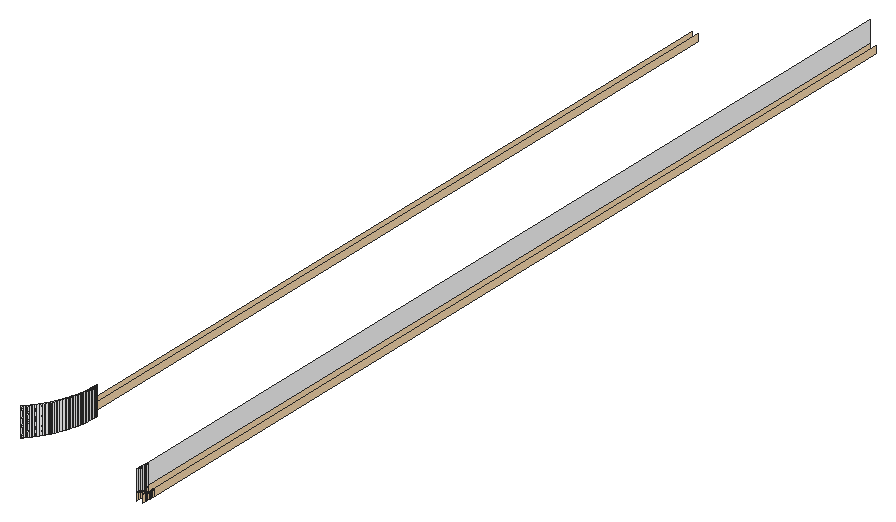
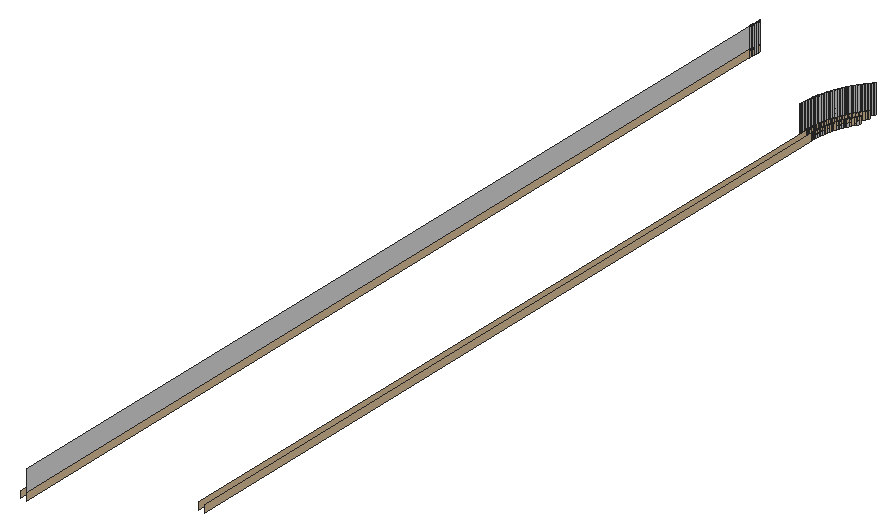
# SketchUp Ruby script. Lengths in inches.
U = 1.inch
M = Sketchup.active_model
def pt(a) = Geom::Point3d.new(a.map { |v| v * U })
def face(e, loops, mat)
  f = e.add_face(loops[0].map { |a| pt(a) })
  loops[1..].each { |l| e.add_face(l.map { |a| pt(a) }).erase! }
  f.material = f.back_material = mat if mat
  f
end
# faces: each face lists its corners as indices into pts; further lists are holes
def faces(e, pts, list, mat = nil) = list.each { |f| face(e, (f[0].is_a?(Array) ? f : [f]).map { |l| l.map { |i| pts[i] } }, mat) }
# xy, xz, yz: faces in a plane at the given z, y or x. An outline is a flat list of corners, or four numbers for a rectangle; further outlines are holes
def ring(l) = l.size == 4 ? [[l[0], l[1]], [l[2], l[1]], [l[2], l[3]], [l[0], l[3]]] : l.each_slice(2).to_a
def flat(e, list, mat, &to3) = list.each { |f| face(e, (f[0].is_a?(Array) ? f : [f]).map { |l| ring(l).map { |u, v| to3.(u, v) } }, mat) }
def xy(e, z, list, mat = nil) = flat(e, list, mat) { |x, y| [x, y, z] }
def xz(e, y, list, mat = nil) = flat(e, list, mat) { |x, z| [x, y, z] }
def yz(e, x, list, mat = nil) = flat(e, list, mat) { |y, z| [x, y, z] }
def lines(e, pts, list) = list.each { |a, b| e.add_line(pt(pts[a]), pt(pts[b])) }
# prism: a flat outline (further loops are holes) pulled along v
def prism(e, loops, v, mat = nil)
  f = face(e, loops, mat); d = Geom::Vector3d.new(v.map { |x| x * U })
  f.pushpull(f.normal.samedirection?(d) ? d.length : -d.length)
end
def box(e, o, s, mat = nil) = prism(e, [[o, [o[0] + s[0], o[1], o[2]], [o[0] + s[0], o[1] + s[1], o[2]], [o[0], o[1] + s[1], o[2]]]], [0, 0, s[2]], mat)
def at(x, y, z, deg = 0) = Geom::Transformation.translation(pt([x, y, z])) * Geom::Transformation.rotation(ORIGIN, Z_AXIS, deg.degrees)
def axes(o, x, y, z) = Geom::Transformation.new([*x, 0, *y, 0, *z, 0, *pt(o).to_a, 1])
def part(name) = M.definitions.add(name)
# library, detail: a bought-in or finely detailed component or shape, given as its bounding box
def library(name, o, s) = part(name).tap { |d| box(d.entities, o, s) }
def detail(e, o, s) = box(e.add_group.entities, o, s)
def put(e, d, t, mat = nil) = e.add_instance(d, t).tap { |i| i.material = mat if mat }
def group(e, t, mat = nil) = e.add_group.tap { |g| g.transformation = t; g.material = mat if mat }.entities
root = M.entities
M.materials.add("False Ceiling Light").color = [254, 223, 179]
M.materials.add("[Quartz Light Grey]").color = [251, 251, 252]
yz(root,178.5,[[77.65,115.32,77.82,116.49],[77.82,115.32,78,116.49],[78,115.32,204,116.49]],"False Ceiling Light")
yz(root,178.5,[[77.65,115.32,77.82,115.91],[77.82,115.32,78,115.91]],"[Quartz Light Grey]")
yz(root,179.5,[[77.62,115.32,77.81,116.49],[77.81,115.32,77.99,116.49],[77.99,115.32,204.01,116.49]],"False Ceiling Light")
yz(root,180.49,[[77.39,115.32,77.59,120]],"[Quartz Light Grey]")
yz(root,180.5,[[77.8,115.32,77.99,120]],"[Quartz Light Grey]")
yz(root,198.5,[[65.55,115.32,65.77,116.49],[65.77,115.32,66.01,116.49],[66.01,115.32,215.99,116.49]],"False Ceiling Light")
yz(root,198.5,[[65.55,115.32,65.77,120],[65.77,115.32,66.01,120],[66.01,115.32,215.99,120]],"[Quartz Light Grey]")
yz(root,199.5,[[65.53,115.32,65.76,116.49],[65.76,115.32,66,116.49],[66,115.32,216,116.49]],"False Ceiling Light")
p = [[198.4,63.98,115.32],[198.38,63.75,115.32],[198.38,63.75,116.49],[198.4,63.98,116.49],[198.38,63.75,115.32],[198.4,63.98,115.32],
  [198.4,63.98,120],[198.38,63.75,120],[199.4,63.88,115.32],[199.42,64.12,115.32],[199.42,64.12,116.49],[199.4,63.88,116.49],
  [198.42,64.2,115.32],[198.42,64.2,116.49],[198.42,64.2,115.32],[198.42,64.2,120],[199.44,64.35,115.32],[199.44,64.35,116.49],
  [198.44,64.43,115.32],[198.44,64.43,116.49],[198.44,64.43,115.32],[198.44,64.43,120],[198.46,64.65,115.32],[198.46,64.65,116.49],
  [198.46,64.65,115.32],[198.46,64.65,120],[199.46,64.59,115.32],[199.46,64.59,116.49],[199.47,64.82,115.32],[199.47,64.82,116.49],
  [198.47,64.875,115.32],[198.47,64.875,116.49],[198.47,64.875,115.32],[198.47,64.875,120],[199.48,65.06,115.32],[199.48,65.06,116.49],
  [198.48,65.1,115.32],[198.48,65.1,116.49],[198.48,65.1,115.32],[198.48,65.1,120],[198.49,65.32,115.32],[198.49,65.32,116.49],
  [198.49,65.32,115.32],[198.49,65.32,120],[199.49,65.29,115.32],[199.49,65.29,116.49],[198.5,65.55,115.32],[198.5,65.55,116.49],
  [198.5,65.55,115.32],[198.5,65.55,120],[199.5,65.53,115.32],[199.5,65.53,116.49],[176.38,67.48,115.32],[176.24,67.33,115.32],
  [176.24,67.33,120],[176.38,67.48,120],[176.52,67.63,115.32],[176.52,67.63,120],[176.65,67.78,115.32],[176.65,67.78,120],
  [176.79,67.93,115.32],[176.79,67.93,120],[176.92,68.09,115.32],[176.92,68.09,120],[177.05,68.25,115.32],[177.05,68.25,120],
  [177.17,68.4,115.32],[177.17,68.4,120],[177.3,68.5625,115.32],[177.3,68.5625,120],[177.42,68.73,115.32],[177.42,68.73,120],
  [176.15,68.73,115.32],[176.27,68.875,115.32],[176.27,68.875,116.49],[176.15,68.73,116.49],[177.54,68.89,115.32],[177.54,68.89,120],
  [176.39,69.02,115.32],[176.39,69.02,116.49],[177.66,69.05,115.32],[177.66,69.05,120],[176.5,69.17,115.32],[176.5,69.17,116.49],
  [177.77,69.22,115.32],[177.77,69.22,120],[176.62,69.32,115.32],[176.62,69.32,116.49],[177.89,69.39,115.32],[177.89,69.39,120],
  [176.73,69.48,115.32],[176.73,69.48,116.49],[178,69.56,115.32],[178,69.56,120],[176.84,69.63,115.32],[176.84,69.63,116.49],
  [176.95,69.79,115.32],[176.95,69.79,116.49],[178.11,69.73,115.32],[178.11,69.73,120],[178.22,69.9,115.32],[178.22,69.9,120],
  [177.06,69.94,115.32],[177.06,69.94,116.49],[177.16,70.1,115.32],[177.16,70.1,116.49],[178.32,70.07,115.32],[178.32,70.07,120],
  [177.26,70.26,115.32],[177.26,70.26,116.49],[178.42,70.25,115.32],[178.42,70.25,120],[178.52,70.43,115.32],[178.52,70.43,120],
  [177.36,70.42,115.32],[177.36,70.42,116.49],[177.46,70.59,115.32],[177.46,70.59,116.49],[178.62,70.6,115.32],[178.62,70.6,120],
  [176.32,70.65,115.32],[176.22,70.5,115.32],[176.22,70.5,116.49],[176.32,70.65,116.49],[176.22,70.5,115.32],[176.32,70.65,115.32],
  [176.32,70.65,115.91],[176.22,70.5,115.91],[176.42,70.8,115.32],[176.42,70.8,116.49],[176.42,70.8,115.32],[176.42,70.8,115.91],
  [177.56,70.75,115.32],[177.56,70.75,116.49],[178.72,70.78,115.32],[178.72,70.78,120],[177.65,70.91,115.32],[177.65,70.91,116.49],
  [176.51,70.95,115.32],[176.51,70.95,116.49],[176.51,70.95,115.32],[176.51,70.95,115.91],[178.8125,70.96,115.32],[178.8125,70.96,120],
  [176.6,71.1,115.32],[176.6,71.1,116.49],[176.6,71.1,115.32],[176.6,71.1,115.91],[177.74,71.08,115.32],[177.74,71.08,116.49],
  [178.9,71.14,115.32],[178.9,71.14,120],[176.69,71.25,115.32],[176.69,71.25,116.49],[176.69,71.25,115.32],[176.69,71.25,115.91],
  [177.83,71.25,115.32],[177.83,71.25,116.49],[178.99,71.33,115.32],[178.99,71.33,120],[176.78,71.4,115.32],[176.78,71.4,116.49],
  [176.78,71.4,115.32],[176.78,71.4,115.91],[177.92,71.42,115.32],[177.92,71.42,116.49],[179.08,71.51,115.32],[179.08,71.51,120],
  [176.86,71.56,115.32],[176.86,71.56,116.49],[176.86,71.56,115.32],[176.86,71.56,115.91],[178,71.59,115.32],[178,71.59,116.49],
  [179.16,71.7,115.32],[179.16,71.7,120],[176.95,71.71,115.32],[176.95,71.71,116.49],[176.95,71.71,115.32],[176.95,71.71,115.91],
  [178.09,71.76,115.32],[178.09,71.76,116.49],[177.03,71.87,115.32],[177.03,71.87,116.49],[177.03,71.87,115.32],[177.03,71.87,115.91],
  [179.24,71.88,115.32],[179.24,71.88,120],[178.17,71.93,115.32],[178.17,71.93,116.49],[177.11,72.03,115.32],[177.11,72.03,116.49],
  [177.11,72.03,115.32],[177.11,72.03,115.91],[178.25,72.1,115.32],[178.25,72.1,116.49],[179.32,72.07,115.32],[179.32,72.07,120],
  [177.18,72.1875,115.32],[177.18,72.1875,116.49],[177.18,72.1875,115.32],[177.18,72.1875,115.91],[178.32,72.28,115.32],[178.32,72.28,116.49],
  [179.4,72.26,115.32],[179.4,72.26,120],[177.26,72.35,115.32],[177.26,72.35,116.49],[177.26,72.35,115.32],[177.26,72.35,115.91],
  [177.33,72.51,115.32],[177.33,72.51,116.49],[177.33,72.51,115.32],[177.33,72.51,115.91],[178.4,72.45,115.32],[178.4,72.45,116.49],
  [179.47,72.45,115.32],[179.47,72.45,120],[179.54,72.64,115.32],[179.54,72.64,120],[177.4,72.67,115.32],[177.4,72.67,116.49],
  [177.4,72.67,115.32],[177.4,72.67,115.91],[178.47,72.625,115.32],[178.47,72.625,116.49],[178.54,72.8,115.32],[178.54,72.8,116.49],
  [179.61,72.83,115.32],[179.61,72.83,120],[177.47,72.83,115.32],[177.47,72.83,116.49],[177.47,72.83,115.32],[177.47,72.83,115.91],
  [177.54,73,115.32],[177.54,73,116.49],[177.54,73,115.32],[177.54,73,115.91],[178.6,72.98,115.32],[178.6,72.98,116.49],
  [179.68,73.02,115.32],[179.68,73.02,120],[177.6,73.16,115.32],[177.6,73.16,116.49],[177.6,73.16,115.32],[177.6,73.16,115.91],
  [178.67,73.16,115.32],[178.67,73.16,116.49],[179.74,73.21,115.32],[179.74,73.21,120],[177.67,73.33,115.32],[177.67,73.33,116.49],
  [177.67,73.33,115.32],[177.67,73.33,115.91],[178.73,73.34,115.32],[178.73,73.34,116.49],[179.8,73.4,115.32],[179.8,73.4,120],
  [177.73,73.49,115.32],[177.73,73.49,116.49],[177.73,73.49,115.32],[177.73,73.49,115.91],[178.79,73.52,115.32],[178.79,73.52,116.49],
  [179.86,73.6,115.32],[179.86,73.6,120],[177.78,73.66,115.32],[177.78,73.66,116.49],[177.78,73.66,115.32],[177.78,73.66,115.91],
  [178.85,73.7,115.32],[178.85,73.7,116.49],[179.92,73.79,115.32],[179.92,73.79,120],[177.84,73.83,115.32],[177.84,73.83,116.49],
  [177.84,73.83,115.32],[177.84,73.83,115.91],[178.9,73.88,115.32],[178.9,73.88,116.49],[177.89,74,115.32],[177.89,74,116.49],
  [177.89,74,115.32],[177.89,74,115.91],[179.97,73.99,115.32],[179.97,73.99,120],[178.96,74.0625,115.32],[178.96,74.0625,116.49],
  [177.94,74.17,115.32],[177.94,74.17,116.49],[177.94,74.17,115.32],[177.94,74.17,115.91],[180.02,74.18,115.32],[180.02,74.18,120],
  [179.01,74.25,115.32],[179.01,74.25,116.49],[177.99,74.34,115.32],[177.99,74.34,116.49],[177.99,74.34,115.32],[177.99,74.34,115.91],
  [179.05,74.43,115.32],[179.05,74.43,116.49],[180.07,74.38,115.32],[180.07,74.38,120],[178.04,74.51,115.32],[178.04,74.51,116.49],
  [178.04,74.51,115.32],[178.04,74.51,115.91],[179.1,74.62,115.32],[179.1,74.62,116.49],[180.12,74.58,115.32],[180.12,74.58,120],
  [178.08,74.68,115.32],[178.08,74.68,116.49],[178.08,74.68,115.32],[178.08,74.68,115.91],[179.14,74.8,115.32],[179.14,74.8,116.49],
  [180.16,74.78,115.32],[180.16,74.78,120],[178.13,74.85,115.32],[178.13,74.85,116.49],[178.13,74.85,115.32],[178.13,74.85,115.91],
  [178.17,75.02,115.32],[178.17,75.02,116.49],[178.17,75.02,115.32],[178.17,75.02,115.91],[179.18,74.99,115.32],[179.18,74.99,116.49],
  [180.2,74.98,115.32],[180.2,74.98,120],[178.21,75.19,115.32],[178.21,75.19,116.49],[178.21,75.19,115.32],[178.21,75.19,115.91],
  [179.22,75.17,115.32],[179.22,75.17,116.49],[180.24,75.18,115.32],[180.24,75.18,120],[178.24,75.37,115.32],[178.24,75.37,116.49],
  [178.24,75.37,115.32],[178.24,75.37,115.91],[179.26,75.36,115.32],[179.26,75.36,116.49],[180.28,75.375,115.32],[180.28,75.375,120],
  [178.27,75.54,115.32],[178.27,75.54,116.49],[178.27,75.54,115.32],[178.27,75.54,115.91],[179.29,75.54,115.32],[179.29,75.54,116.49],
  [180.31,75.58,115.32],[180.31,75.58,120],[178.31,75.71,115.32],[178.31,75.71,116.49],[178.31,75.71,115.32],[178.31,75.71,115.91],
  [179.32,75.73,115.32],[179.32,75.73,116.49],[180.34,75.78,115.32],[180.34,75.78,120],[178.33,75.89,115.32],[178.33,75.89,116.49],
  [178.33,75.89,115.32],[178.33,75.89,115.91],[179.35,75.92,115.32],[179.35,75.92,116.49],[180.37,75.98,115.32],[180.37,75.98,120],
  [178.36,76.0625,115.32],[178.36,76.0625,116.49],[178.36,76.0625,115.32],[178.36,76.0625,115.91],[179.375,76.11,115.32],[179.375,76.11,116.49],
  [180.39,76.18,115.32],[180.39,76.18,120],[178.38,76.24,115.32],[178.38,76.24,116.49],[178.38,76.24,115.32],[178.38,76.24,115.91],
  [179.4,76.3,115.32],[179.4,76.3,116.49],[178.41,76.41,115.32],[178.41,76.41,116.49],[178.41,76.41,115.32],[178.41,76.41,115.91],
  [180.42,76.38,115.32],[180.42,76.38,120],[179.42,76.48,115.32],[179.42,76.48,116.49],[178.43,76.59,115.32],[178.43,76.59,116.49],
  [178.43,76.59,115.32],[178.43,76.59,115.91],[180.44,76.58,115.32],[180.44,76.58,120],[179.4375,76.67,115.32],[179.4375,76.67,116.49],
  [178.44,76.76,115.32],[178.44,76.76,116.49],[178.44,76.76,115.32],[178.44,76.76,115.91],[180.45,76.78,115.32],[180.45,76.78,120],
  [179.46,76.86,115.32],[179.46,76.86,116.49],[178.46,76.94,115.32],[178.46,76.94,116.49],[178.46,76.94,115.32],[178.46,76.94,115.91],
  [180.47,76.99,115.32],[180.47,76.99,120],[178.47,77.12,115.32],[178.47,77.12,116.49],[178.47,77.12,115.32],[178.47,77.12,115.91],
  [179.47,77.05,115.32],[179.47,77.05,116.49],[180.48,77.1875,115.32],[180.48,77.1875,120],[178.48,77.29,115.32],[178.48,77.29,116.49],
  [178.48,77.29,115.32],[178.48,77.29,115.91],[179.48,77.24,115.32],[179.48,77.24,116.49],[179.49,77.43,115.32],[179.49,77.43,116.49],
  [180.49,77.39,115.32],[180.49,77.39,120],[178.49,77.47,115.32],[178.49,77.47,116.49],[178.49,77.47,115.32],[178.49,77.47,115.91],
  [179.5,77.62,115.32],[179.5,77.62,116.49],[178.5,77.65,115.32],[178.5,77.65,116.49],[178.5,77.65,115.32],[178.5,77.65,115.91],
  [180.5,77.8,115.32],[180.49,77.59,115.32],[180.49,77.59,120],[180.5,77.8,120],[177,66.0625,120],[177,66,120],
  [176.9375,66,120]]
faces(root,p,[[0,1,2,3],[8,9,10,11],[12,0,3,13],[9,16,17,10],[18,12,13,19],[22,18,19,23],[16,26,27,17],[26,28,29,27],
  [30,22,23,31],[28,34,35,29],[36,30,31,37],[40,36,37,41],[34,44,45,35],[46,40,41,47],[44,50,51,45],[72,73,74,75],
  [73,78,79,74],[78,82,83,79],[82,86,87,83],[86,90,91,87],[90,94,95,91],[94,96,97,95],[96,102,103,97],[102,104,105,103],
  [104,108,109,105],[108,114,115,109],[114,116,117,115],[120,121,122,123],[128,120,123,129],[116,132,133,117],[132,136,137,133],[138,128,129,139],
  [144,138,139,145],[136,148,149,137],[152,144,145,153],[148,156,157,149],[160,152,153,161],[156,164,165,157],[168,160,161,169],[164,172,173,165],
  [176,168,169,177],[172,180,181,173],[182,176,177,183],[180,188,189,181],[190,182,183,191],[188,194,195,189],[198,190,191,199],[194,202,203,195],
  [206,198,199,207],[210,206,207,211],[202,214,215,203],[220,210,211,221],[214,224,225,215],[224,226,227,225],[230,220,221,231],[234,230,231,235],
  [226,238,239,227],[242,234,235,243],[238,246,247,239],[250,242,243,251],[246,254,255,247],[258,250,251,259],[254,262,263,255],[266,258,259,267],
  [262,270,271,263],[274,266,267,275],[270,278,279,271],[280,274,275,281],[278,286,287,279],[288,280,281,289],[286,294,295,287],[296,288,289,297],
  [294,300,301,295],[304,296,297,305],[300,308,309,301],[312,304,305,313],[308,316,317,309],[320,312,313,321],[324,320,321,325],[316,328,329,317],
  [332,324,325,333],[328,336,337,329],[340,332,333,341],[336,344,345,337],[348,340,341,349],[344,352,353,345],[356,348,349,357],[352,360,361,353],
  [364,356,357,365],[360,368,369,361],[372,364,365,373],[368,376,377,369],[380,372,373,381],[376,384,385,377],[386,380,381,387],[384,392,393,385],
  [394,386,387,395],[392,400,401,393],[402,394,395,403],[400,408,409,401],[410,402,403,411],[416,410,411,417],[408,420,421,409],[424,416,417,425],
  [420,428,429,421],[428,430,431,429],[434,424,425,435],[430,438,439,431],[440,434,435,441]],"False Ceiling Light")
faces(root,p,[[4,5,6,7],[5,14,15,6],[14,20,21,15],[20,24,25,21],[24,32,33,25],[32,38,39,33],[38,42,43,39],[42,48,49,43],
  [52,53,54,55],[56,52,55,57],[58,56,57,59],[60,58,59,61],[62,60,61,63],[64,62,63,65],[66,64,65,67],[68,66,67,69],
  [70,68,69,71],[76,70,71,77],[80,76,77,81],[84,80,81,85],[88,84,85,89],[92,88,89,93],[98,92,93,99],[100,98,99,101],
  [106,100,101,107],[110,106,107,111],[112,110,111,113],[118,112,113,119],[124,125,126,127],[125,130,131,126],[134,118,119,135],[130,140,141,131],
  [142,134,135,143],[140,146,147,141],[150,142,143,151],[146,154,155,147],[158,150,151,159],[154,162,163,155],[166,158,159,167],[162,170,171,163],
  [174,166,167,175],[170,178,179,171],[178,184,185,179],[186,174,175,187],[184,192,193,185],[196,186,187,197],[192,200,201,193],[204,196,197,205],
  [200,208,209,201],[208,212,213,209],[216,204,205,217],[218,216,217,219],[212,222,223,213],[228,218,219,229],[222,232,233,223],[232,236,237,233],
  [240,228,229,241],[236,244,245,237],[248,240,241,249],[244,252,253,245],[256,248,249,257],[252,260,261,253],[264,256,257,265],[260,268,269,261],
  [272,264,265,273],[268,276,277,269],[276,282,283,277],[284,272,273,285],[282,290,291,283],[292,284,285,293],[290,298,299,291],[302,292,293,303],
  [298,306,307,299],[310,302,303,311],[306,314,315,307],[318,310,311,319],[314,322,323,315],[322,326,327,323],[330,318,319,331],[326,334,335,327],
  [338,330,331,339],[334,342,343,335],[346,338,339,347],[342,350,351,343],[354,346,347,355],[350,358,359,351],[362,354,355,363],[358,366,367,359],
  [370,362,363,371],[366,374,375,367],[378,370,371,379],[374,382,383,375],[382,388,389,383],[390,378,379,391],[388,396,397,389],[398,390,391,399],
  [396,404,405,397],[406,398,399,407],[404,412,413,405],[414,406,407,415],[412,418,419,413],[422,414,415,423],[418,426,427,419],[432,422,423,433],
  [426,436,437,427],[436,442,443,437],[444,445,446,447]],"[Quartz Light Grey]")
lines(root,p,[[448,449],[449,450]])
